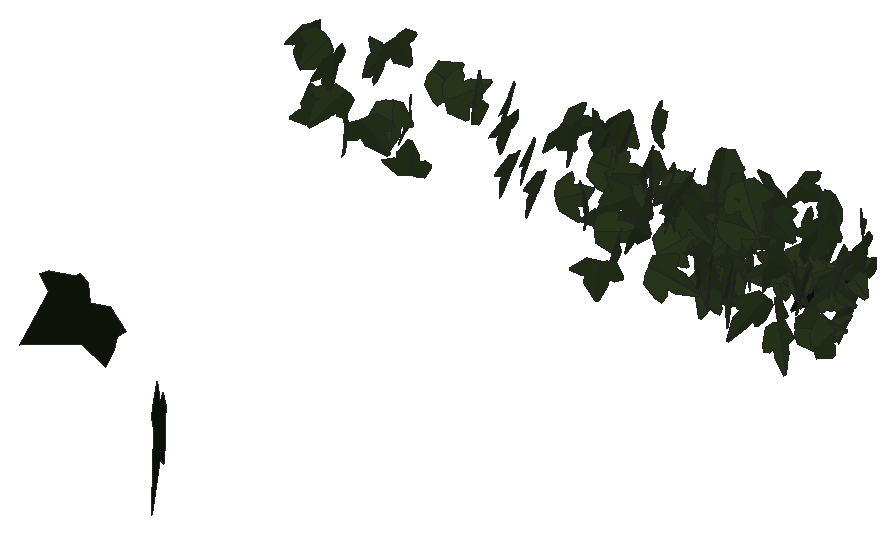
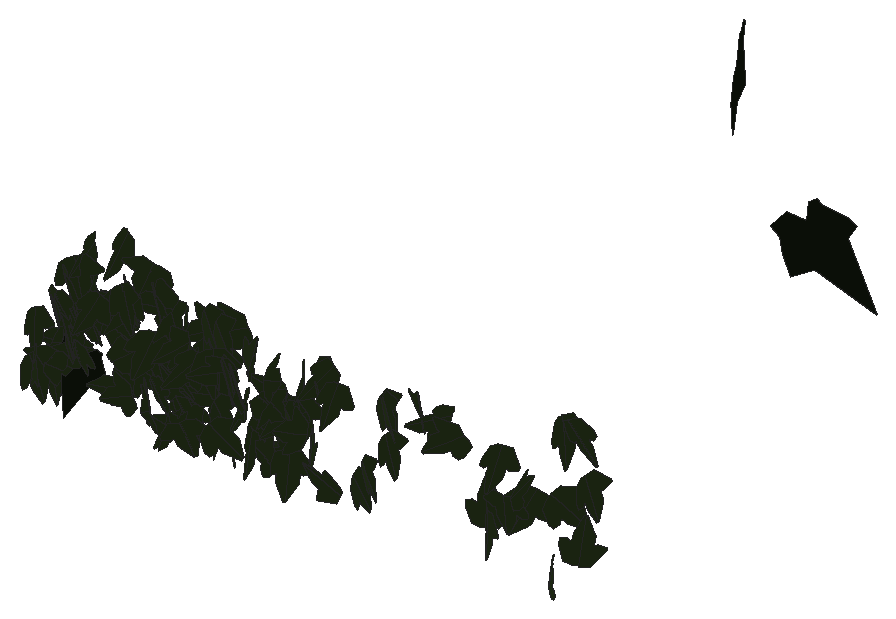
# SketchUp Ruby script. Lengths in inches.
U = 1.inch
M = Sketchup.active_model
def pt(a) = Geom::Point3d.new(a.map { |v| v * U })
def face(e, loops, mat)
  f = e.add_face(loops[0].map { |a| pt(a) })
  loops[1..].each { |l| e.add_face(l.map { |a| pt(a) }).erase! }
  f.material = f.back_material = mat if mat
  f
end
# faces: each face lists its corners as indices into pts; further lists are holes
def faces(e, pts, list, mat = nil) = list.each { |f| face(e, (f[0].is_a?(Array) ? f : [f]).map { |l| l.map { |i| pts[i] } }, mat) }
# xy, xz, yz: faces in a plane at the given z, y or x. An outline is a flat list of corners, or four numbers for a rectangle; further outlines are holes
def ring(l) = l.size == 4 ? [[l[0], l[1]], [l[2], l[1]], [l[2], l[3]], [l[0], l[3]]] : l.each_slice(2).to_a
def flat(e, list, mat, &to3) = list.each { |f| face(e, (f[0].is_a?(Array) ? f : [f]).map { |l| ring(l).map { |u, v| to3.(u, v) } }, mat) }
def xy(e, z, list, mat = nil) = flat(e, list, mat) { |x, y| [x, y, z] }
def xz(e, y, list, mat = nil) = flat(e, list, mat) { |x, z| [x, y, z] }
def yz(e, x, list, mat = nil) = flat(e, list, mat) { |y, z| [x, y, z] }
def lines(e, pts, list) = list.each { |a, b| e.add_line(pt(pts[a]), pt(pts[b])) }
# prism: a flat outline (further loops are holes) pulled along v
def prism(e, loops, v, mat = nil)
  f = face(e, loops, mat); d = Geom::Vector3d.new(v.map { |x| x * U })
  f.pushpull(f.normal.samedirection?(d) ? d.length : -d.length)
end
def box(e, o, s, mat = nil) = prism(e, [[o, [o[0] + s[0], o[1], o[2]], [o[0] + s[0], o[1] + s[1], o[2]], [o[0], o[1] + s[1], o[2]]]], [0, 0, s[2]], mat)
def at(x, y, z, deg = 0) = Geom::Transformation.translation(pt([x, y, z])) * Geom::Transformation.rotation(ORIGIN, Z_AXIS, deg.degrees)
def axes(o, x, y, z) = Geom::Transformation.new([*x, 0, *y, 0, *z, 0, *pt(o).to_a, 1])
def part(name) = M.definitions.add(name)
# library, detail: a bought-in or finely detailed component or shape, given as its bounding box
def library(name, o, s) = part(name).tap { |d| box(d.entities, o, s) }
def detail(e, o, s) = box(e.add_group.entities, o, s)
def put(e, d, t, mat = nil) = e.add_instance(d, t).tap { |i| i.material = mat if mat }
def group(e, t, mat = nil) = e.add_group.tap { |g| g.transformation = t; g.material = mat if mat }.entities
root = M.entities
M.materials.add("efeu1").color = [18, 25, 13]
M.materials.add("efeu2").color = [43, 57, 29]
c1 = part("ivyleaf_10")
p = [[0,0.5,-0.03],[-0.0625,2.02,-0.43],[-0.19,2.01,-0.46],[-0.54,1.05,-0.29],[-0.52,0.625,-0.18],[-0.83,0.76,-0.28],
  [-1.16,0.64,-0.33],[-1.15,0.33,-0.24],[-0.77,-0.39,0.02],[-0.3,-0.51,0.16],[0.04,-0.48,0.23],[-0.02,2.01,-0.4375],
  [-0.06,2.01,-0.43],[0.04,-0.49,0.23],[0.67,-0.49,0.14],[1.38,0.36,-0.2],[1.375,0.51,-0.24],[0.81,0.65,-0.19],
  [0.62,0.59,-0.15],[0.6,1.09,-0.28],[0.5,1.23,-0.31]]
faces(c1.entities,p,[[0,1,2,3,4,5,6,7,8,9,10],[11,12,0,13,14,15,16,17,18,19,20]],"efeu2")
c2 = part("ivyleaf_9")
p = [[1.54,2.16,1.25],[1.36,2.04,1.19],[-0.21,0.99,0.68],[-0.71,1.11,0.82],[-0.85,0.86,0.67],[-0.8,0.17,0.21],
  [-0.9,-0.01,0.1],[-0.67,-0.16,-0.02],[-0.08,-0.08,-0.05],[-0.03,-0.6,-0.4],[0.65,-0.88,-0.66],[0.83,-0.6,-0.49],
  [1.29,-0.42,-0.43],[1.8125,-0.07,-0.26],[1.21,0.44,0.15]]
faces(c2.entities,p,[[0,1,2,3,4,5,6,7,8,9,10,11,12,13,14]],"efeu1")
put(root,c1,axes([496.68,137.51,152.0625],[-0.05368,-0.66898,0.10962],[-0.00948,-0.10921,-0.67113],[0.67783,-0.05451,-0.00071]))
put(root,c1,axes([497.1875,137.34,149.11],[-0.41001,-0.5067,-0.17803],[-0.11045,-0.13963,0.6518],[-0.52558,0.42462,0.0019]))
put(root,c1,axes([497.73,138.21,148.24],[0.026,-0.02956,0.63621],[0.48292,-0.41422,-0.03898],[0.41523,0.48359,0.0055]))
put(root,c1,axes([498.54,136.77,150.45],[-0.27652,-0.41447,0.49617],[-0.21709,-0.44879,-0.49588],[0.60897,-0.34819,0.04853]))
put(root,c1,axes([498.54,135.86,152.89],[0.58101,-0.18765,-0.37464],[-0.35672,0.11448,-0.61056],[0.21981,0.68178,-0.00059]))
put(root,c1,axes([498.95,138.49,151.33],[-0.12695,0.01373,0.63664],[0.28204,-0.58081,0.06877],[0.57092,0.28998,0.10759]))
put(root,c1,axes([499.1875,135.66,152.64],[-0.01489,-0.72101,-0.11407],[0.00959,0.11389,-0.72113],[0.72992,-0.01621,0.00714]))
put(root,c1,axes([499.93,138.22,152.42],[-0.22607,-0.55517,-0.29055],[0.13548,0.25826,-0.5989],[0.61178,-0.26234,0.02526]))
put(root,c1,axes([499.96,136.52,149.97],[-0.57476,-0.29866,-0.31656],[0.27278,0.16139,-0.64753],[0.33912,-0.63601,-0.01566]))
put(root,c1,axes([500.39,138.23,149.75],[0.14918,-0.45395,-0.49396],[-0.14847,0.47114,-0.47781],[0.65423,0.21043,0.0042]))
put(root,c1,axes([500.22,137.52,150.19],[0.67312,0.07528,0.08797],[0.08694,0.01412,-0.6773],[-0.07647,0.6787,0.00433]))
put(root,c2,axes([502.35,118.52,151.8],[0.23598,0.15867,-1.22816],[-1.01204,-0.71868,-0.28074],[-0.79483,0.96219,-0.00717]))
put(root,c1,axes([501.66,136.77,148.77],[-0.61039,-0.28412,0.00304],[0.01452,-0.024,0.6727],[-0.28377,0.60992,0.02788]))
put(root,c1,axes([502.17,137.75,152.06],[0.31999,0.20168,0.61131],[0.52718,0.30965,-0.37811],[-0.3694,0.61661,-0.01007]))
put(root,c1,axes([503.35,137.01,152.07],[0.2059,-0.03249,-0.68031],[0.39819,0.58234,0.0927],[0.55255,-0.40755,0.18669]))
put(root,c1,axes([504.35,136.96,151.8],[0.54248,-0.3464,0.26823],[-0.22502,0.14599,0.64365],[-0.3759,-0.5873,0.00179]))
put(root,c1,axes([504.79,138.16,151.1],[0.02648,-0.6428,0.04508],[0.00001,-0.04512,-0.64335],[0.64438,0.02642,-0.00184]))
put(root,c1,axes([505.09,137.875,152.35],[0.27398,-0.59078,0.0055],[0.0017,-0.00527,-0.65121],[0.5908,0.27398,-0.00067]))
put(root,c1,axes([505.41,138.56,150.0625],[0.28517,-0.56001,0.1104],[0.04647,-0.10023,-0.62843],[0.5689,0.2889,-0.00401]))
put(root,c1,axes([506,138.29,149.22],[0.17501,-0.581,0.25946],[0.08665,-0.24482,-0.60668],[0.63037,0.19496,0.01136]))
put(root,c1,axes([506.56,136.13,151.09],[0.15316,-0.63183,0.17339],[0.03841,-0.1691,-0.65012],[0.65406,0.15789,-0.00243]))
put(root,c1,axes([506.9,138.56,148.76],[0.29169,-0.13408,-0.57663],[0.57154,-0.10381,0.31326],[-0.15435,-0.63781,0.07023]))
put(root,c1,axes([507.48,137.65,151.9],[-0.20532,-0.52572,-0.32906],[0.11979,0.30648,-0.5644],[0.60854,-0.23771,0.00007]))
put(root,c1,axes([507.76,139.28,150.93],[0.09709,-0.3198,0.55072],[-0.0705,0.54826,0.3308],[-0.63292,-0.11013,0.04764]))
put(root,c1,axes([507.95,137.47,152.43],[-0.12539,-0.28147,-0.60718],[0.24521,0.55546,-0.30813],[0.62271,-0.27541,-0.00092]))
put(root,c1,axes([508.28,137.52,152.33],[0.2185,-0.54931,0.2742],[0.1412,-0.23828,-0.58987],[0.59748,0.2572,0.03912]))
put(root,c1,axes([508.33,139.02,151.31],[0.31534,-0.56584,0.18487],[0.0772,-0.16857,-0.64763],[0.59025,0.32435,-0.01406]))
put(root,c1,axes([508.22,138.02,149.04],[-0.28955,0.23475,0.54766],[0.4264,-0.34368,0.37275],[0.4162,0.51542,-0.00088]))
put(root,c1,axes([508.45,138.24,152.4375],[-0.2101,0.48136,-0.37522],[0.10932,-0.36073,-0.52399],[-0.60046,-0.23411,0.03589]))
put(root,c1,axes([508.86,139.3125,151.68],[0.07718,0.49273,-0.40019],[-0.07253,-0.39365,-0.49867],[-0.63061,0.10559,0.00838]))
put(root,c1,axes([509.12,138.15,148.93],[-0.61756,-0.32765,0.00284],[-0.00234,-0.00163,-0.6991],[0.32765,-0.61757,0.00034]))
put(root,c1,axes([508.74,138.2,150.8125],[0.14265,0.31111,0.6065],[0.26369,0.54621,-0.34221],[-0.62857,0.29974,-0.00591]))
put(root,c1,axes([509.36,138.87,152.25],[0.09286,-0.30136,0.60915],[0.33701,-0.51348,-0.3054],[0.59018,0.34062,0.07855]))
put(root,c1,axes([509.35,138.95,149.25],[-0.05696,-0.11281,0.64975],[0.6376,-0.176,0.02534],[0.16844,0.62805,0.1238]))
put(root,c1,axes([509.37,137.625,148.73],[0.09452,-0.04771,-0.64398],[0.62368,0.17544,0.07854],[0.16738,-0.62679,0.071]))
put(root,c1,axes([510.35,137.61,150.33],[-0.31729,-0.1209,0.5577],[-0.51593,-0.21191,-0.33946],[0.24386,-0.60564,0.00745]))
put(root,c1,axes([510.2,137.98,150.78],[0.45795,0.12814,-0.46823],[-0.45243,-0.1207,-0.47552],[-0.17599,0.64373,0.00404]))
put(root,c1,axes([510.16,137.17,148.34],[0.26262,-0.28417,0.55907],[-0.33393,0.44969,0.38543],[-0.53085,-0.42345,0.03413]))
put(root,c1,axes([509.69,140.03,151.875],[0.30708,-0.30845,-0.46453],[0.31923,-0.33756,0.43517],[-0.45719,-0.44287,-0.00815]))
put(root,c1,axes([510.27,138.64,149.57],[0.09085,-0.50518,-0.45873],[-0.05082,0.45648,-0.51277],[0.68048,0.10154,0.02295]))
put(root,c1,axes([509.89,137.75,151.125],[0.1358,-0.02568,-0.62399],[0.61291,-0.11708,0.1382],[-0.11986,-0.62777,-0.00025]))
put(root,c1,axes([510.3,139.125,151.125],[-0.10651,0.54055,-0.34534],[0.067,-0.33878,-0.55094],[-0.63794,-0.12583,-0.0002]))
put(root,c2,axes([509.9,112.95,152.82],[-0.13378,0.08012,-1.30407],[1.21395,-0.55599,-0.15243],[-0.60641,-1.13071,-0.01745]))
put(root,c1,axes([510.89,139.84,150.17],[-0.30168,-0.34945,0.45715],[-0.30326,-0.3421,-0.46163],[0.48901,-0.42774,-0.00426]))
put(root,c1,axes([510.89,137.48,149.48],[-0.00509,-0.47896,-0.49731],[0.00813,0.49725,-0.47899],[0.69041,-0.00939,0.00197]))
put(root,c1,axes([511.11,135.16,148.99],[-0.59483,-0.38718,0.09762],[-0.08155,-0.05366,-0.70974],[0.39088,-0.6004,0.00048]))
put(root,c1,axes([511.08,137.82,151.84],[-0.04206,-0.11947,-0.66552],[0.14972,-0.65189,0.10756],[-0.65937,-0.14041,0.06688]))
put(root,c1,axes([511.71,138.64,150.21],[0.0702,-0.59789,0.21849],[0.0506,-0.21388,-0.60152],[0.63455,0.0832,0.0238]))
put(root,c1,axes([511.87,138.09,151.46],[0.35284,-0.55596,-0.04211],[-0.02253,0.03558,-0.65847],[0.55709,0.35356,0.00004]))
put(root,c1,axes([511.76,138.66,148.82],[-0.33532,0.13904,0.55531],[0.3905,-0.41503,0.33971],[0.41859,0.49856,0.12793]))
put(root,c1,axes([512.19,137.4,147.99],[0.48607,-0.27392,0.41375],[-0.35958,0.20469,0.55794],[-0.34195,-0.60461,0.00143]))
put(root,c1,axes([512.61,137.31,150.6],[0.17423,-0.57237,-0.44109],[-0.11771,0.42519,-0.59823],[0.71296,0.21008,0.00903]))
put(root,c1,axes([512.05,137.86,151.2],[-0.15138,-0.09888,-0.63937],[0.62022,0.16469,-0.17232],[0.18412,-0.63607,0.05477]))
put(root,c1,axes([512.68,137.74,151.41],[-0.49794,-0.43541,0.05291],[-0.03924,-0.0355,-0.66145],[0.43685,-0.49948,0.00089]))
put(root,c1,axes([512.66,139.38,149.49],[0.5209,0.35059,-0.16954],[-0.14047,-0.09492,-0.62789],[-0.36322,0.5395,-0.0003]))
put(root,c1,axes([512.66,137.43,149.88],[-0.09843,-0.04671,-0.70152],[0.70295,0.00683,-0.09909],[0.01327,-0.70836,0.0453]))
put(root,c1,axes([513.23,136.65,151.86],[0.21724,-0.6449,0.15211],[0.0444,-0.14555,-0.68049],[0.66111,0.22169,-0.00428]))
put(root,c1,axes([513.37,137.02,151.52],[0.21785,-0.64846,0.29497],[0.09143,-0.28045,-0.68407],[0.7065,0.23625,-0.00243]))
put(root,c1,axes([513.48,136.99,152.35],[0.1894,-0.64026,0.08217],[0.01948,-0.07993,-0.66767],[0.64522,0.19036,-0.00397]))
put(root,c1,axes([513.33,138.01,151.12],[-0.16988,-0.2444,-0.60156],[0.30741,0.51743,-0.29703],[0.57193,-0.35071,-0.01903]))
put(root,c1,axes([513.42,137.17,151.03],[-0.59515,0.42501,-0.17549],[0.14238,-0.10259,-0.73133],[-0.43721,-0.61194,0.00072]))
put(root,c1,axes([513.61,138.34,151.85],[0.00253,0.00823,0.65497],[-0.07514,0.65065,-0.00789],[-0.65069,-0.0751,0.00345]))
put(root,c1,axes([513.72,138.6,148.59],[0.01751,0.5523,-0.32851],[-0.00869,0.3288,0.55233],[0.64255,-0.0106,0.01642]))
put(root,c1,axes([513.375,135.94,150.22],[0.3871,0.01827,-0.54213],[0.51061,0.21252,0.37175],[0.18309,-0.63134,0.10945]))
put(root,c1,axes([513.69,137.74,148.61],[-0.46779,-0.05026,0.4431],[0.44347,0.01509,0.46989],[-0.04689,0.64415,0.02356]))
put(root,c1,axes([514.02,138.28,152.82],[0.06309,0.64123,-0.31004],[-0.06331,-0.30497,-0.64364],[-0.70943,0.08424,0.02987]))
put(root,c1,axes([514.05,137.32,150.18],[-0.10301,0.09852,0.6633],[0.222,-0.62823,0.12779],[0.63277,0.23644,0.06315]))
put(root,c1,axes([513.82,139.75,149.87],[0.3054,-0.10631,0.59024],[0.54318,-0.23178,-0.32279],[0.25426,0.62284,-0.01938]))
put(root,c1,axes([513.75,136.41,151.61],[0.36231,0.00679,0.65215],[0.64339,0.11836,-0.35868],[-0.10673,0.73658,0.05162]))
put(root,c1,axes([514.27,137.1,148.71],[0.66127,0.04672,-0.04449],[-0.04485,0.00365,-0.66288],[-0.04637,0.66275,0.00678]))
put(root,c1,axes([514.06,137.63,149.49],[0.48531,-0.1457,-0.42236],[0.42446,-0.04429,0.503],[-0.13946,-0.64183,0.06117]))
put(root,c1,axes([514.35,137.81,148.18],[0.16127,0.38769,-0.48276],[0.19581,0.44133,0.41983],[0.58739,-0.25356,-0.00741]))
put(root,c1,axes([514.6,137.07,149.28],[0.52877,-0.48718,0.12363],[0.09403,-0.08039,-0.71897],[0.49374,0.53705,0.00452]))
put(root,c1,axes([514.54,136.23,149.625],[-0.31342,0.28867,0.50802],[0.37473,-0.34302,0.4261],[0.44832,0.48853,-0.001]))
put(root,c1,axes([515.32,137.6,150.32],[0.27039,0.0986,0.58055],[-0.5729,-0.10371,0.28443],[0.1362,-0.63198,0.0439]))
put(root,c1,axes([514.47,140.14,150.42],[0.25072,-0.00362,0.59161],[0.58323,0.10933,-0.24651],[-0.09927,0.63317,0.04594]))
put(root,c1,axes([514.46,134.14,150.41],[0.21281,0.14576,0.7096],[0.58783,0.39748,-0.25794],[-0.42336,0.62516,-0.00146]))
put(root,c1,axes([514.98,138.22,151.48],[-0.48299,-0.41566,-0.28145],[0.21145,0.18578,-0.63722],[0.45528,-0.52724,-0.00264]))
put(root,c1,axes([515.35,137.44,149.32],[0.41597,-0.30166,-0.43247],[-0.34834,0.25632,-0.51383],[0.39585,0.54255,0.0023]))
put(root,c1,axes([514.86,138.53,149.05],[0.08547,-0.18588,-0.63532],[0.32724,-0.54498,0.20348],[-0.57541,-0.33754,0.02135]))
put(root,c1,axes([515.36,136.89,149.31],[0.60613,-0.02355,-0.29756],[-0.29739,0.01021,-0.60659],[0.02564,0.67515,-0.0012]))
put(root,c1,axes([515.32,137.43,152.7],[0.53545,-0.34827,0.22096],[0.18487,-0.12102,-0.63875],[0.36869,0.56647,-0.00062]))
put(root,c1,axes([515.0625,136.125,149.2],[0.00522,-0.07878,0.72989],[0.72202,0.13257,0.00915],[-0.13279,0.71777,0.07842]))
put(root,c1,axes([515.99,138.47,150.6],[0.14606,0.31587,0.61204],[-0.28926,-0.53967,0.34754],[0.62506,-0.32355,0.01782]))
put(root,c1,axes([515.58,135.52,150.41],[0.28476,-0.25308,0.5701],[0.43691,-0.36634,-0.38086],[0.44516,0.52144,0.00913]))
put(root,c1,axes([516.45,137.91,152.67],[-0.54177,0.07274,0.41151],[-0.40856,0.04941,-0.54662],[-0.08783,-0.67854,0.00431]))
put(root,c1,axes([515.67,136.38,151.78],[0.02022,0.03301,0.75523],[0.67948,0.33031,-0.03263],[-0.3313,0.67946,-0.02083]))
put(root,c1,axes([515.98,136.07,150.21],[0.00488,-0.19008,0.68278],[0.46664,-0.51305,-0.14617],[0.53345,0.45054,0.12161]))
put(root,c1,axes([516.2,135.91,149.89],[0.5042,-0.41362,0.3634],[0.29706,-0.21051,-0.65176],[0.46356,0.58478,0.02241]))
put(root,c1,axes([516,138.375,149.38],[0.00109,-0.01802,0.64676],[0.54314,0.3515,0.00888],[-0.35161,0.54291,0.01572]))
put(root,c1,axes([516.26,136.5625,153.11],[0.6277,0.25171,0.32357],[0.30333,0.11286,-0.67625],[-0.27576,0.69711,-0.00735]))
put(root,c1,axes([516.95,136.42,149.03],[-0.10856,-0.51345,0.55651],[-0.10881,-0.54578,-0.52479],[0.74933,-0.15364,0.00442]))
put(root,c1,axes([516.57,137.19,151.51],[0.35133,-0.39385,-0.43661],[0.27865,-0.33635,0.52764],[-0.51778,-0.44825,-0.01229]))
put(root,c1,axes([516.9,138.8,152.57],[-0.22653,-0.3895,-0.44968],[0.21799,0.39336,-0.45054],[0.55354,-0.31431,-0.0066]))
put(root,c1,axes([516.93,137.23,152.03],[-0.39155,-0.42383,-0.35869],[0.25972,0.24813,-0.5767],[0.49075,-0.46947,0.01902]))
put(root,c1,axes([517.56,136.77,150.45],[0.37067,-0.02856,-0.60696],[-0.60264,0.07369,-0.3715],[0.07775,0.70737,0.0142]))
put(root,c1,axes([518.34,138.83,152.13],[0.31887,-0.23708,-0.51009],[-0.41009,0.30335,-0.39735],[0.385,0.51947,-0.00077]))
put(root,c1,axes([518.31,140.3125,150.55],[0.05457,-0.1307,-0.62812],[-0.21765,0.58923,-0.14152],[0.60353,0.22431,0.00576]))
put(root,c1,axes([518.43,138.59,151.44],[0.29324,-0.38266,-0.5931],[-0.36607,0.46666,-0.48208],[0.60347,0.46902,-0.00423]))
put(root,c2,axes([518.38,137.6,149.49],[0.26512,0.7127,0.07502],[0.02484,0.0708,-0.76042],[-0.71621,0.26628,0.00139]))
put(root,c1,axes([518.12,137.34,150.27],[0.5794,-0.27175,-0.14039],[0.12802,-0.05766,0.63996],[-0.2778,-0.59337,0.0021]))
put(root,c1,axes([518.36,138.08,150.69],[-0.13151,0.04158,0.65408],[0.11504,-0.65529,0.06479],[0.64522,0.12531,0.12176]))
put(root,c1,axes([518.26,135.85,149.66],[-0.22744,0.52827,-0.27261],[0.10835,-0.25015,-0.57515],[-0.5845,-0.25193,-0.00054]))
put(root,c1,axes([518.37,137.94,149.99],[0.66774,-0.28628,0.03483],[0.03201,-0.01373,-0.72652],[0.28661,0.66851,0]))
put(root,c1,axes([518.56,136.26,150.88],[-0.53784,0.44317,0.1226],[-0.09925,0.07233,-0.69686],[-0.44897,-0.54687,0.00718]))
put(root,c1,axes([518,136.68,150.51],[0.23554,-0.03678,0.64673],[0.64109,-0.08536,-0.23835],[0.09282,0.68297,0.00504]))
put(root,c1,axes([518.46,138.32,152.67],[0.54507,-0.43776,0.08882],[0.0736,-0.0502,-0.69906],[0.44057,0.54998,0.00689]))
put(root,c1,axes([518.66,138.75,149.73],[-0.08147,-0.36708,0.52453],[-0.07527,-0.51961,-0.37532],[0.63578,-0.10856,0.02278]))
put(root,c1,axes([518.39,136.62,151.1],[0.48947,0.51408,0.11966],[0.0826,0.08658,-0.70982],[-0.52132,0.49639,-0.00011]))
put(root,c1,axes([518.52,138.09,150.46],[0.24005,-0.57595,0.31996],[0.15655,-0.28092,-0.62313],[0.63999,0.28475,0.03242]))
put(root,c1,axes([518.32,136.52,150.99],[0.0157,-0.16133,-0.69699],[0.60645,0.37285,-0.07264],[0.37954,-0.58909,0.14491]))
put(root,c1,axes([518.99,139.54,149.82],[-0.08523,-0.70397,0.12732],[-0.02038,-0.12578,-0.70909],[0.7151,-0.08749,-0.00504]))
put(root,c1,axes([518.65,138.96,150],[0.35218,0.40626,0.36962],[0.24598,0.27592,-0.53764],[-0.49108,0.42955,-0.00423]))
put(root,c1,axes([519.18,137.04,152.43],[-0.48499,-0.44035,0.12962],[-0.08743,-0.0965,-0.65496],[0.45063,-0.49265,0.01243]))
put(root,c1,axes([519.21,137.82,149.85],[0.17634,0.25187,-0.58998],[-0.3337,-0.48655,-0.30745],[-0.54787,0.37742,-0.00263]))
put(root,c1,axes([519.07,134.51,152.28],[0.01207,-0.43341,-0.60314],[0.08435,0.60012,-0.42955],[0.73791,-0.06151,0.05897]))
put(root,c1,axes([518.75,136.74,148.59],[0.01025,-0.01031,0.67258],[0.4217,0.52415,0.00161],[-0.52405,0.42158,0.01444]))
put(root,c1,axes([519.24,136.1,152.625],[0.02931,-0.14677,-0.75612],[0.01937,0.75657,-0.1461],[0.76999,-0.01345,0.03246]))
put(root,c1,axes([519.38,138.03,148.89],[0.03699,-0.64776,-0.02521],[0.00037,0.02527,-0.64881],[0.64825,0.03694,0.00181]))
put(root,c1,axes([518.78,137.79,149.93],[0.11443,-0.04758,0.69596],[0.69405,0.07871,-0.10873],[-0.07017,0.7009,0.05946]))
put(root,c1,axes([519.04,134.86,149.41],[0.57798,-0.10428,0.39461],[0.38764,-0.0739,-0.5873],[0.12777,0.69593,-0.00323]))
put(root,c1,axes([519.47,138.81,151.13],[-0.00417,-0.63198,-0.20325],[-0.00132,0.20326,-0.63199],[0.66386,-0.00356,-0.00253]))
put(root,c1,axes([519.35,136.04,151.22],[0.3606,-0.56197,0.19686],[0.10235,-0.16822,-0.6677],[0.58659,0.37481,-0.00452]))
put(root,c1,axes([519.35,136.78,148.32],[0.08453,0.20682,-0.66335],[0.27989,0.6015,0.2232],[0.63599,-0.2922,-0.01006]))
put(root,c1,axes([519.68,137.58,151.18],[0.41069,-0.58027,-0.08719],[-0.05067,0.07095,-0.7109],[0.58459,0.4138,-0.00037]))
